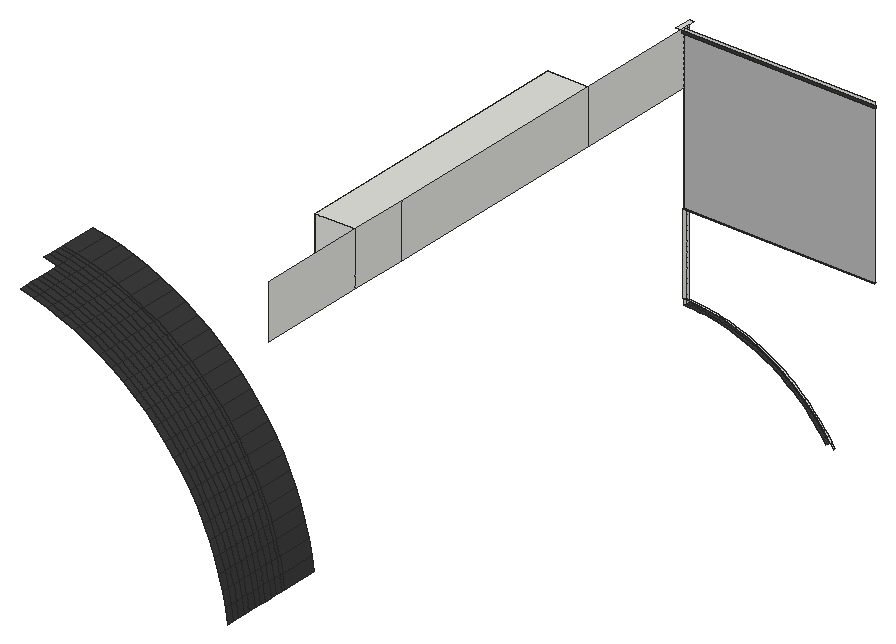
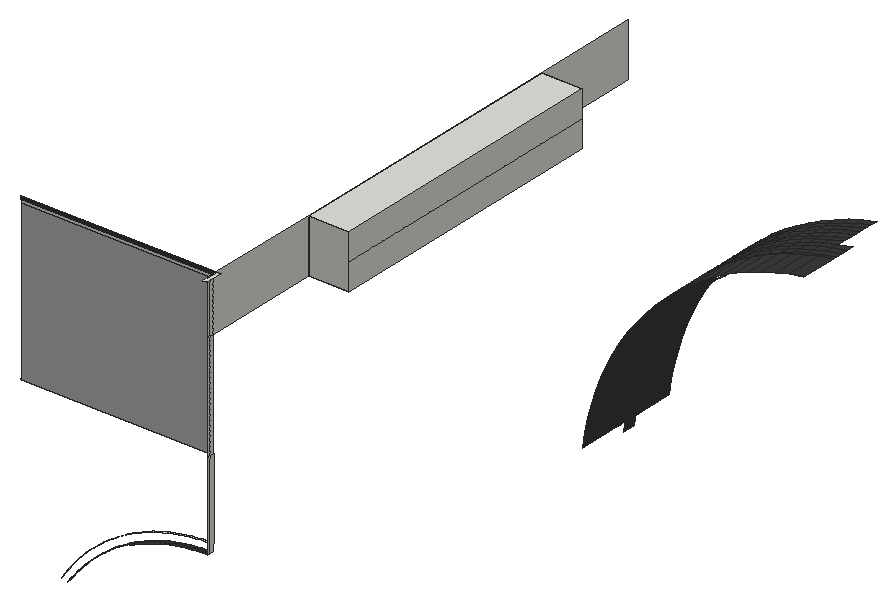
# SketchUp Ruby script. Lengths in inches.
U = 1.inch
M = Sketchup.active_model
def pt(a) = Geom::Point3d.new(a.map { |v| v * U })
def face(e, loops, mat)
  f = e.add_face(loops[0].map { |a| pt(a) })
  loops[1..].each { |l| e.add_face(l.map { |a| pt(a) }).erase! }
  f.material = f.back_material = mat if mat
  f
end
# faces: each face lists its corners as indices into pts; further lists are holes
def faces(e, pts, list, mat = nil) = list.each { |f| face(e, (f[0].is_a?(Array) ? f : [f]).map { |l| l.map { |i| pts[i] } }, mat) }
# xy, xz, yz: faces in a plane at the given z, y or x. An outline is a flat list of corners, or four numbers for a rectangle; further outlines are holes
def ring(l) = l.size == 4 ? [[l[0], l[1]], [l[2], l[1]], [l[2], l[3]], [l[0], l[3]]] : l.each_slice(2).to_a
def flat(e, list, mat, &to3) = list.each { |f| face(e, (f[0].is_a?(Array) ? f : [f]).map { |l| ring(l).map { |u, v| to3.(u, v) } }, mat) }
def xy(e, z, list, mat = nil) = flat(e, list, mat) { |x, y| [x, y, z] }
def xz(e, y, list, mat = nil) = flat(e, list, mat) { |x, z| [x, y, z] }
def yz(e, x, list, mat = nil) = flat(e, list, mat) { |y, z| [x, y, z] }
def lines(e, pts, list) = list.each { |a, b| e.add_line(pt(pts[a]), pt(pts[b])) }
# prism: a flat outline (further loops are holes) pulled along v
def prism(e, loops, v, mat = nil)
  f = face(e, loops, mat); d = Geom::Vector3d.new(v.map { |x| x * U })
  f.pushpull(f.normal.samedirection?(d) ? d.length : -d.length)
end
def box(e, o, s, mat = nil) = prism(e, [[o, [o[0] + s[0], o[1], o[2]], [o[0] + s[0], o[1] + s[1], o[2]], [o[0], o[1] + s[1], o[2]]]], [0, 0, s[2]], mat)
def at(x, y, z, deg = 0) = Geom::Transformation.translation(pt([x, y, z])) * Geom::Transformation.rotation(ORIGIN, Z_AXIS, deg.degrees)
def axes(o, x, y, z) = Geom::Transformation.new([*x, 0, *y, 0, *z, 0, *pt(o).to_a, 1])
def part(name) = M.definitions.add(name)
# library, detail: a bought-in or finely detailed component or shape, given as its bounding box
def library(name, o, s) = part(name).tap { |d| box(d.entities, o, s) }
def detail(e, o, s) = box(e.add_group.entities, o, s)
def put(e, d, t, mat = nil) = e.add_instance(d, t).tap { |i| i.material = mat if mat }
def group(e, t, mat = nil) = e.add_group.tap { |g| g.transformation = t; g.material = mat if mat }.entities
root = M.entities
M.materials.add("[Color M07]").color = [58, 58, 58]
M.materials.add("[Mirror 01]").color = [185, 185, 185]
xy(root,331.79,[[154.46,115.33,156.04,115.71]])
xy(root,349.6875,[[154.46,115.33,197.34,115.71]])
xy(root,373.6875,[[145.46,24,154.46,88.96]])
xy(root,385.6875,[[145.46,24,154.46,88.96],[153.51,114.76,154.46,118.4375]])
xz(root,24,[[145.46,373.6875,154.46,385.6875]])
xz(root,88.96,[[145.46,373.6875,154.46,385.6875]])
xz(root,114.76,[[154.46,385.0625,197.91,385.6875]],"[Color M07]")
xz(root,115.71,[[154.46,385.0625,196.96,385.6875]])
xz(root,115.71,[[154.46,349.6875,196.96,385.0625]],"[Mirror 01]")
yz(root,145.46,[[24,373.6875,88.96,379.6875],[24,379.6875,88.96,385.6875]])
yz(root,154.46,[[115.71,330.25,116.39,330.25,116.39,349.6875,115.33,349.6875,115.33,331.79,115.71,331.79],[116.39,330.25,117.08,349.6875],[115.71,349.6875,116.39,373.6875],[116.39,349.6875,117.08,373.6875],[0,373.6875,24,385.6875],
  [24,373.6875,37.13,385.6875],[37.13,373.6875,88.96,385.6875],[88.96,373.6875,115.71,373.6875,115.71,385.0625,114.76,385.0625,114.76,385.6875,88.96,385.6875],[115.71,373.6875,116.39,385.0625],[116.39,373.6875,117.08,385.0625],
  [114.76,385.0625,115.71,385.6875],[115.71,385.0625,116.39,385.6875],[116.39,385.0625,117.08,385.6875]])
p = [[187.43,115.71,314.375],[188.12,115.71,313.33],[188.12,115.33,313.33],[187.43,115.33,314.375],[185.43,115.71,314.47],[185.43,116.39,314.47],
  [186.12,116.39,313.49],[186.12,115.71,313.49],[143.06,14.875,316.87],[143.51,14.875,313.82],[143.51,12,313.82],[143.06,12,316.87],
  [144.86,0,317.1875],[144.86,1.5,317.1875],[145.32,1.5,314.03],[145.32,0,314.03],[144.86,3,317.1875],[145.32,3,314.03],
  [144.86,4.5,317.1875],[145.32,4.5,314.03],[144.86,6,317.1875],[145.32,6,314.03],[144.86,7.5,317.1875],[145.32,7.5,314.03],
  [144.86,9,317.1875],[145.32,9,314.03],[144.86,10.5,317.1875],[145.32,10.5,314.03],[144.86,12,317.1875],[145.32,12,314.03],
  [144.86,13.5,317.1875],[145.32,13.5,314.03],[144.86,15,317.1875],[145.32,15,314.03],[144.86,15.8125,317.1875],[145.32,15.8125,314.03],
  [145.32,24,314.03],[144.86,24,317.1875],[186.71,115.71,315.4],[186.71,115.33,315.4],[184.71,115.71,315.43],[184.71,116.39,315.43],
  [185.96,115.71,316.4],[185.96,115.33,316.4],[183.96,115.71,316.37],[183.96,116.39,316.37],[185.17,115.71,317.375],[185.17,115.33,317.375],
  [183.18,115.71,317.28],[183.18,116.39,317.28],[142.44,14.875,319.9],[142.44,12,319.9],[144.22,0,320.31],[144.22,1.5,320.31],
  [144.22,3,320.31],[144.22,4.5,320.31],[144.22,6,320.31],[144.22,7.5,320.31],[144.22,9,320.31],[144.22,10.5,320.31],
  [144.22,12,320.31],[144.22,13.5,320.31],[144.22,15,320.31],[144.22,15.8125,320.31],[144.22,24,320.31],[182.37,115.71,318.17],
  [182.37,116.39,318.17],[184.36,115.71,318.33],[184.36,115.33,318.33],[181.53,115.71,319.04],[181.53,116.39,319.04],[183.52,115.71,319.26],
  [183.52,115.33,319.26],[180.67,115.71,319.875],[180.67,116.39,319.875],[182.65,115.71,320.15],[182.65,115.33,320.15],[141.67,14.875,322.89],
  [141.67,12,322.89],[179.78,115.71,320.68],[179.78,116.39,320.68],[181.75,115.71,321.03],[181.75,115.33,321.03],[143.42,0,323.39],
  [143.42,1.5,323.39],[143.42,3,323.39],[143.42,4.5,323.39],[143.42,6,323.39],[143.42,7.5,323.39],[143.42,9,323.39],
  [143.42,10.5,323.39],[143.42,12,323.39],[143.42,13.5,323.39],[143.42,15,323.39],[143.42,15.8125,323.39],[143.42,24,323.39],
  [178.86,115.71,321.46],[178.86,116.39,321.46],[180.82,115.71,321.87],[180.82,115.33,321.87],[177.92,115.71,322.22],[177.92,116.39,322.22],
  [179.87,115.71,322.68],[179.87,115.33,322.68],[176.96,115.71,322.9375],[176.96,116.39,322.9375],[178.89,115.71,323.46],[178.89,115.33,323.46],
  [140.73,14.875,325.83],[140.73,12,325.83],[175.98,115.71,323.63],[175.98,116.39,323.63],[142.46,0,326.43],[142.46,1.5,326.43],
  [142.46,3,326.43],[142.46,4.5,326.43],[142.46,6,326.43],[142.46,7.5,326.43],[142.46,9,326.43],[142.46,10.5,326.43],
  [142.46,12,326.43],[142.46,13.5,326.43],[142.46,15,326.43],[142.46,15.8125,326.43],[142.46,24,326.43],[177.89,115.71,324.22],
  [177.89,115.33,324.22],[174.97,115.71,324.29],[174.97,116.39,324.29],[176.87,115.71,324.9375],[176.87,115.33,324.9375],[173.95,115.71,324.92],
  [173.95,116.39,324.92],[175.82,115.71,325.625],[175.82,115.33,325.625],[172.9,115.71,325.51],[172.9,116.39,325.51],[171.84,115.71,326.08],
  [171.84,116.39,326.08],[174.75,115.71,326.28],[174.75,115.33,326.28],[139.64,14.875,328.72],[139.64,12,328.72],[170.76,115.71,326.61],
  [170.76,116.39,326.61],[170.76,117.08,326.61],[171.84,117.08,326.08],[173.66,115.71,326.9],[173.66,115.33,326.9],[141.33,0,329.41],
  [141.33,1.5,329.41],[141.33,3,329.41],[141.33,4.5,329.41],[141.33,6,329.41],[141.33,7.5,329.41],[141.33,9,329.41],
  [141.33,10.5,329.41],[141.33,12,329.41],[141.33,13.5,329.41],[141.33,15,329.41],[141.33,15.8125,329.41],[141.33,24,329.41],
  [169.66,115.71,327.1],[169.66,116.39,327.1],[169.66,117.08,327.1],[172.56,115.71,327.49],[172.56,115.33,327.49],[168.55,115.71,327.5625],
  [168.55,116.39,327.5625],[168.55,117.08,327.5625],[171.43,115.71,328.04],[171.43,115.33,328.04],[167.43,115.71,327.99],[167.43,116.39,327.99],
  [167.43,117.08,327.99],[170.29,115.71,328.55],[170.29,115.33,328.55],[166.29,115.71,328.375],[166.29,116.39,328.375],[166.29,117.08,328.375],
  [165.14,115.71,328.73],[165.14,116.39,328.73],[165.14,117.08,328.73],[169.13,115.71,329.03],[169.13,115.33,329.03],[138.39,14.875,331.54],
  [138.39,12,331.54],[163.98,115.71,329.05],[163.98,116.39,329.05],[163.98,117.08,329.05],[167.96,115.71,329.47],[167.96,115.33,329.47],
  [162.8125,115.71,329.33],[162.8125,116.39,329.33],[162.8125,117.08,329.33],[161.63,115.71,329.57],[161.63,116.39,329.57],[161.63,117.08,329.57],
  [140.05,0,332.33],[140.05,1.5,332.33],[140.05,3,332.33],[140.05,4.5,332.33],[140.05,6,332.33],[140.05,7.5,332.33],
  [140.05,9,332.33],[140.05,10.5,332.33],[140.05,12,332.33],[140.05,13.5,332.33],[140.05,15,332.33],[140.05,15.8125,332.33],
  [140.05,24,332.33],[166.78,115.71,329.88],[166.78,115.33,329.88],[160.45,115.71,329.78],[160.45,116.39,329.78],[160.45,117.08,329.78],
  [159.26,115.71,329.95],[159.26,116.39,329.95],[159.26,117.08,329.95],[165.58,115.71,330.25],[165.58,115.33,330.25],[158.0625,115.71,330.08],
  [158.0625,116.39,330.08],[158.0625,117.08,330.08],[156.86,115.71,330.17],[156.86,116.39,330.17],[156.86,117.08,330.17],[164.375,115.71,330.58],
  [164.375,115.33,330.58],[154.46,115.71,330.25],[154.46,116.39,330.25],[155.66,116.39,330.23],[155.66,115.71,330.23],[154.46,117.08,330.25],
  [155.66,117.08,330.23],[163.16,115.71,330.87],[163.16,115.33,330.87],[161.93,115.71,331.125],[161.93,115.33,331.125],[160.7,115.71,331.34],
  [160.7,115.33,331.34],[159.46,115.71,331.52],[159.46,115.33,331.52],[137,14.875,334.3],[137,12,334.3],[158.21,115.71,331.65],
  [158.21,115.33,331.65],[156.96,115.71,331.75],[156.96,115.33,331.75],[156.04,115.71,331.79],[156.04,115.33,331.79],[138.61,0,335.17],
  [138.61,1.5,335.17],[138.61,3,335.17],[138.61,4.5,335.17],[138.61,6,335.17],[138.61,7.5,335.17],[138.61,9,335.17],
  [138.61,10.5,335.17],[138.61,12,335.17],[138.61,13.5,335.17],[138.61,15,335.17],[138.61,15.8125,335.17],[138.61,24,335.17],
  [135.46,14.875,336.97],[135.46,12,336.97],[137.02,0,337.93],[137.02,1.5,337.93],[137.02,3,337.93],[137.02,4.5,337.93],
  [137.02,6,337.93],[137.02,7.5,337.93],[137.02,9,337.93],[137.02,10.5,337.93],[137.02,12,337.93],[137.02,13.5,337.93],
  [137.02,15,337.93],[137.02,15.8125,337.93],[137.02,24,337.93],[133.77,14.875,339.5625],[133.77,12,339.5625],[135.28,0,340.6],
  [135.28,1.5,340.6],[135.28,3,340.6],[135.28,4.5,340.6],[135.28,6,340.6],[135.28,7.5,340.6],[135.28,9,340.6],
  [135.28,10.5,340.6],[135.28,12,340.6],[135.28,13.5,340.6],[135.28,15,340.6],[135.28,15.8125,340.6],[135.28,24,340.6],
  [131.95,14.875,342.06],[131.95,12,342.06],[133.4,0,343.17],[133.4,1.5,343.17],[133.4,3,343.17],[133.4,4.5,343.17],
  [133.4,6,343.17],[133.4,7.5,343.17],[133.4,9,343.17],[133.4,10.5,343.17],[133.4,12,343.17],[133.4,13.5,343.17],
  [133.4,15,343.17],[133.4,15.8125,343.17],[133.4,24,343.17],[130,14.875,344.45],[130,12,344.45],[131.39,0,345.64],
  [131.39,1.5,345.64],[131.39,3,345.64],[131.39,4.5,345.64],[131.39,6,345.64],[131.39,7.5,345.64],[131.39,9,345.64],
  [131.39,10.5,345.64],[131.39,12,345.64],[131.39,13.5,345.64],[131.39,15,345.64],[131.39,15.8125,345.64],[131.39,24,345.64],
  [127.93,14.875,346.74],[127.93,12,346.74],[129.25,0,348],[129.25,1.5,348],[129.25,3,348],[129.25,4.5,348],
  [129.25,6,348],[129.25,7.5,348],[129.25,9,348],[129.25,10.5,348],[129.25,12,348],[129.25,13.5,348],
  [129.25,15,348],[129.25,15.8125,348],[129.25,24,348],[125.73,14.875,348.91],[125.73,12,348.91],[126.98,0,350.24],
  [126.98,1.5,350.24],[126.98,3,350.24],[126.98,4.5,350.24],[126.98,6,350.24],[126.98,7.5,350.24],[126.98,9,350.24],
  [126.98,10.5,350.24],[126.98,12,350.24],[126.98,13.5,350.24],[126.98,15,350.24],[126.98,15.8125,350.24],[126.98,24,350.24],
  [123.42,14.875,350.95],[123.42,12,350.95],[124.6,0,352.36],[124.6,1.5,352.36],[124.6,3,352.36],[124.6,4.5,352.36],
  [124.6,6,352.36],[124.6,7.5,352.36],[124.6,9,352.36],[124.6,10.5,352.36],[124.6,12,352.36],[124.6,13.5,352.36],
  [124.6,15,352.36],[124.6,15.8125,352.36],[124.6,24,352.36],[121,14.875,352.875],[121,12,352.875],[122.1,0,354.34],
  [122.1,1.5,354.34],[122.1,3,354.34],[122.1,4.5,354.34],[122.1,6,354.34],[122.1,7.5,354.34],[122.1,9,354.34],
  [122.1,10.5,354.34],[122.1,12,354.34],[122.1,13.5,354.34],[122.1,15,354.34],[122.1,15.8125,354.34],[122.1,24,354.34],
  [118.49,14.875,354.67],[118.49,12,354.67],[119.51,0,356.1875],[119.51,1.5,356.1875],[119.51,3,356.1875],[119.51,4.5,356.1875],
  [119.51,6,356.1875],[119.51,7.5,356.1875],[119.51,9,356.1875],[119.51,10.5,356.1875],[119.51,12,356.1875],[119.51,13.5,356.1875],
  [119.51,15,356.1875],[119.51,15.8125,356.1875],[119.51,24,356.1875],[115.88,14.875,356.32],[115.88,12,356.32],[116.81,0,357.89],
  [116.81,1.5,357.89],[116.81,3,357.89],[116.81,4.5,357.89],[116.81,6,357.89],[116.81,7.5,357.89],[116.81,9,357.89],
  [116.81,10.5,357.89],[116.81,12,357.89],[116.81,13.5,357.89],[116.81,15,357.89],[116.81,15.8125,357.89],[116.81,24,357.89],
  [113.18,14.875,357.83],[113.18,12,357.83],[110.41,14.875,359.19],[110.41,12,359.19],[114.04,0,359.45],[114.04,1.5,359.45],
  [114.04,3,359.45],[114.04,4.5,359.45],[114.04,6,359.45],[114.04,7.5,359.45],[114.04,9,359.45],[114.04,10.5,359.45],
  [114.04,12,359.45],[114.04,13.5,359.45],[114.04,15,359.45],[114.04,15.8125,359.45],[114.04,24,359.45],[107.57,14.875,360.4],
  [107.57,12,360.4],[111.18,0,360.85],[111.18,1.5,360.85],[111.18,3,360.85],[111.18,4.5,360.85],[111.18,6,360.85],
  [111.18,7.5,360.85],[111.18,9,360.85],[111.18,10.5,360.85],[111.18,12,360.85],[111.18,13.5,360.85],[111.18,15,360.85],
  [111.18,15.8125,360.85],[111.18,24,360.85],[108.24,0,362.1],[108.24,1.5,362.1],[108.24,3,362.1],[108.24,4.5,362.1],
  [108.24,6,362.1],[108.24,7.5,362.1],[108.24,9,362.1],[108.24,10.5,362.1],[108.24,12,362.1],[104.67,14.875,361.46],
  [106.12,14.875,360.93],[106.12,12,360.93],[104.67,12,361.46],[108.24,13.5,362.1],[108.24,15,362.1],[108.24,15.8125,362.1],
  [108.24,24,362.1],[101.72,14.875,362.36],[101.72,12,362.36],[105.25,0,363.19],[105.25,1.5,363.19],[105.25,3,363.19],
  [105.25,4.5,363.19],[105.25,6,363.19],[105.25,7.5,363.19],[105.25,9,363.19],[105.25,10.5,363.19],[105.25,12,363.19],
  [105.25,13.5,363.19],[105.25,15,363.19],[105.25,15.8125,363.19],[105.25,24,363.19],[98.72,14.875,363.1],[98.72,12,363.1],
  [102.2,0,364.12],[102.2,1.5,364.12],[102.2,3,364.12],[102.2,4.5,364.12],[102.2,6,364.12],[102.2,7.5,364.12],
  [102.2,9,364.12],[102.2,10.5,364.12],[102.2,12,364.12],[102.2,13.5,364.12],[102.2,15,364.12],[102.2,15.8125,364.12],
  [102.2,24,364.12],[99.11,0,364.88],[99.11,1.5,364.88],[99.11,3,364.88],[99.11,4.5,364.88],[99.11,6,364.88],
  [99.11,7.5,364.88],[99.11,9,364.88],[99.11,10.5,364.88],[99.11,12,364.88],[99.11,13.5,364.88],[99.11,15,364.88],
  [99.11,15.8125,364.88],[99.11,24,364.88],[95.98,10.5,365.48],[95.98,12,365.48],[95.98,13.5,365.48],[95.98,15,365.48],
  [95.98,15.8125,365.48],[95.98,24,365.48]]
faces(root,p,[[0,1,2,3],[38,0,3,39],[42,38,39,43],[46,42,43,47],[67,46,47,68],[71,67,68,72],[75,71,72,76],[81,75,76,82],
  [98,81,82,99],[102,98,99,103],[106,102,103,107],[125,106,107,126],[129,125,126,130],[133,129,130,134],[139,133,134,140],[147,139,140,148],
  [165,147,148,166],[170,165,166,171],[175,170,171,176],[183,175,176,184],[190,183,184,191],[211,190,191,212],[219,211,212,220],[227,219,220,228],
  [235,227,228,236],[237,235,236,238],[239,237,238,240],[241,239,240,242],[245,241,242,246],[247,245,246,248],[249,247,248,250]])
faces(root,p,[[4,5,6,7],[8,9,10,11],[12,13,14,15],[13,16,17,14],[16,18,19,17],[18,20,21,19],[20,22,23,21],[22,24,25,23],
  [24,26,27,25],[26,28,29,27],[30,28,29,31],[32,30,31,33],[34,35,33,32],[36,35,34,37],[40,41,5,4],[44,45,41,40],
  [48,49,45,44],[50,8,11,51],[52,53,13,12],[53,54,16,13],[54,55,18,16],[55,56,20,18],[56,57,22,20],[57,58,24,22],
  [58,59,26,24],[59,60,28,26],[61,60,28,30],[62,61,30,32],[63,34,32,62],[37,34,63,64],[65,66,49,48],[69,70,66,65],
  [73,74,70,69],[77,50,51,78],[79,80,74,73],[83,84,53,52],[84,85,54,53],[85,86,55,54],[86,87,56,55],[87,88,57,56],
  [88,89,58,57],[89,90,59,58],[90,91,60,59],[92,91,60,61],[93,92,61,62],[94,63,62,93],[64,63,94,95],[96,97,80,79],
  [100,101,97,96],[104,105,101,100],[108,77,78,109],[110,111,105,104],[112,113,84,83],[113,114,85,84],[114,115,86,85],[115,116,87,86],
  [116,117,88,87],[117,118,89,88],[118,119,90,89],[119,120,91,90],[121,120,91,92],[122,121,92,93],[123,94,93,122],[95,94,123,124],
  [127,128,111,110],[131,132,128,127],[135,136,132,131],[137,138,136,135],[141,108,109,142],[143,144,138,137],[144,145,146,138],[149,150,113,112],
  [150,151,114,113],[151,152,115,114],[152,153,116,115],[153,154,117,116],[154,155,118,117],[155,156,119,118],[156,157,120,119],[158,157,120,121],
  [159,158,121,122],[160,123,122,159],[124,123,160,161],[162,163,144,143],[163,164,145,144],[167,168,163,162],[168,169,164,163],[172,173,168,167],
  [173,174,169,168],[177,178,173,172],[178,179,174,173],[180,181,178,177],[181,182,179,178],[185,141,142,186],[187,188,181,180],[188,189,182,181],
  [192,193,188,187],[193,194,189,188],[195,196,193,192],[196,197,194,193],[198,199,150,149],[199,200,151,150],[200,201,152,151],[201,202,153,152],
  [202,203,154,153],[203,204,155,154],[204,205,156,155],[205,206,157,156],[207,206,157,158],[208,207,158,159],[209,160,159,208],[161,160,209,210],
  [213,214,196,195],[214,215,197,196],[216,217,214,213],[217,218,215,214],[221,222,217,216],[222,223,218,217],[224,225,222,221],[225,226,223,222],
  [229,230,231,232],[232,231,225,224],[230,233,234,231],[231,234,226,225],[243,185,186,244],[251,252,199,198],[252,253,200,199],[253,254,201,200],
  [254,255,202,201],[255,256,203,202],[256,257,204,203],[257,258,205,204],[258,259,206,205],[260,259,206,207],[261,260,207,208],[262,209,208,261],
  [210,209,262,263],[264,243,244,265],[266,267,252,251],[267,268,253,252],[268,269,254,253],[269,270,255,254],[270,271,256,255],[271,272,257,256],
  [272,273,258,257],[273,274,259,258],[275,274,259,260],[276,275,260,261],[277,262,261,276],[263,262,277,278],[279,264,265,280],[281,282,267,266],
  [282,283,268,267],[283,284,269,268],[284,285,270,269],[285,286,271,270],[286,287,272,271],[287,288,273,272],[288,289,274,273],[290,289,274,275],
  [291,290,275,276],[292,277,276,291],[278,277,292,293],[294,279,280,295],[296,297,282,281],[297,298,283,282],[298,299,284,283],[299,300,285,284],
  [300,301,286,285],[301,302,287,286],[302,303,288,287],[303,304,289,288],[305,304,289,290],[306,305,290,291],[307,292,291,306],[293,292,307,308],
  [309,294,295,310],[311,312,297,296],[312,313,298,297],[313,314,299,298],[314,315,300,299],[315,316,301,300],[316,317,302,301],[317,318,303,302],
  [318,319,304,303],[320,319,304,305],[321,320,305,306],[322,307,306,321],[308,307,322,323],[324,309,310,325],[326,327,312,311],[327,328,313,312],
  [328,329,314,313],[329,330,315,314],[330,331,316,315],[331,332,317,316],[332,333,318,317],[333,334,319,318],[335,334,319,320],[336,335,320,321],
  [337,322,321,336],[323,322,337,338],[339,324,325,340],[341,342,327,326],[342,343,328,327],[343,344,329,328],[344,345,330,329],[345,346,331,330],
  [346,347,332,331],[347,348,333,332],[348,349,334,333],[350,349,334,335],[351,350,335,336],[352,337,336,351],[338,337,352,353],[354,339,340,355],
  [356,357,342,341],[357,358,343,342],[358,359,344,343],[359,360,345,344],[360,361,346,345],[361,362,347,346],[362,363,348,347],[363,364,349,348],
  [365,364,349,350],[366,365,350,351],[367,352,351,366],[353,352,367,368],[369,354,355,370],[371,372,357,356],[372,373,358,357],[373,374,359,358],
  [374,375,360,359],[375,376,361,360],[376,377,362,361],[377,378,363,362],[378,379,364,363],[380,379,364,365],[381,380,365,366],[382,367,366,381],
  [368,367,382,383],[384,369,370,385],[386,387,372,371],[387,388,373,372],[388,389,374,373],[389,390,375,374],[390,391,376,375],[391,392,377,376],
  [392,393,378,377],[393,394,379,378],[395,394,379,380],[396,395,380,381],[397,382,381,396],[383,382,397,398],[399,384,385,400],[401,402,387,386],
  [402,403,388,387],[403,404,389,388],[404,405,390,389],[405,406,391,390],[406,407,392,391],[407,408,393,392],[408,409,394,393],[410,409,394,395],
  [411,410,395,396],[412,397,396,411],[398,397,412,413],[414,399,400,415],[416,414,415,417],[418,419,402,401],[419,420,403,402],[420,421,404,403],
  [421,422,405,404],[422,423,406,405],[423,424,407,406],[424,425,408,407],[425,426,409,408],[427,426,409,410],[428,427,410,411],[429,412,411,428],
  [413,412,429,430],[431,416,417,432],[433,434,419,418],[434,435,420,419],[435,436,421,420],[436,437,422,421],[437,438,423,422],[438,439,424,423],
  [439,440,425,424],[440,441,426,425],[442,441,426,427],[443,442,427,428],[444,429,428,443],[430,429,444,445],[446,447,434,433],[447,448,435,434],
  [448,449,436,435],[449,450,437,436],[450,451,438,437],[451,452,439,438],[452,453,440,439],[453,454,441,440],[455,456,457,458],[459,454,441,442],
  [460,459,442,443],[461,444,443,460],[445,444,461,462],[463,455,458,464],[465,466,447,446],[466,467,448,447],[467,468,449,448],[468,469,450,449],
  [469,470,451,450],[470,471,452,451],[471,472,453,452],[472,473,454,453],[474,473,454,459],[475,474,459,460],[476,461,460,475],[462,461,476,477],
  [478,463,464,479],[480,481,466,465],[481,482,467,466],[482,483,468,467],[483,484,469,468],[484,485,470,469],[485,486,471,470],[486,487,472,471],
  [487,488,473,472],[489,488,473,474],[490,489,474,475],[491,476,475,490],[477,476,491,492],[493,494,481,480],[494,495,482,481],[495,496,483,482],
  [496,497,484,483],[497,498,485,484],[498,499,486,485],[499,500,487,486],[500,501,488,487],[502,501,488,489],[503,502,489,490],[504,491,490,503],
  [492,491,504,505],[506,507,501,500],[508,507,501,502],[509,508,502,503],[510,504,503,509],[505,504,510,511]],"[Color M07]")
